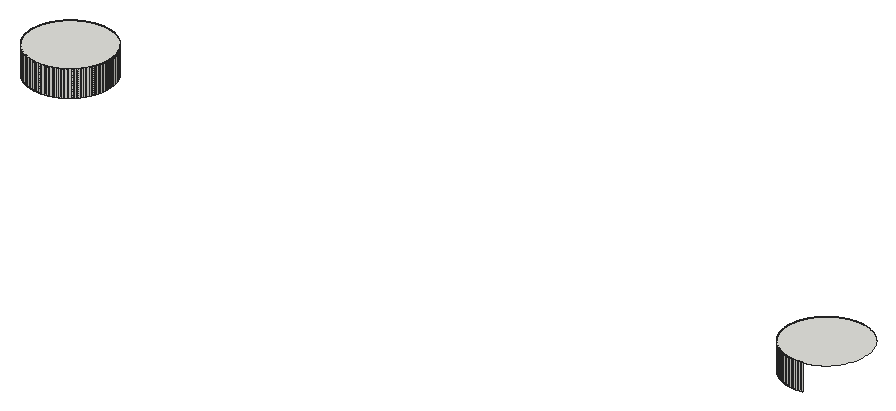
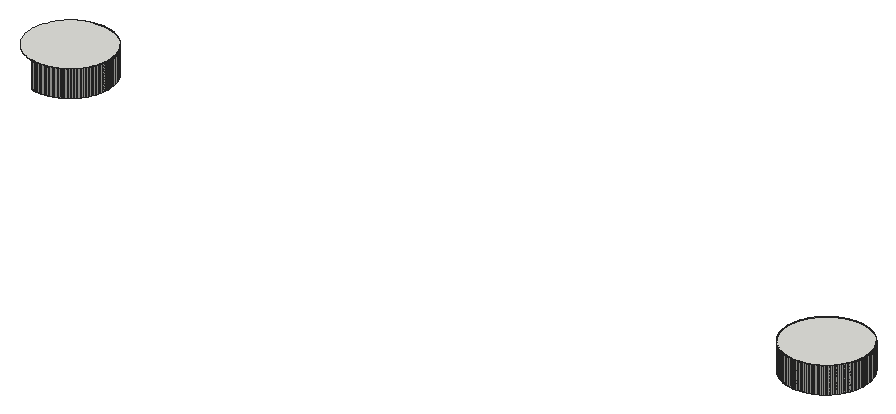
# SketchUp Ruby script. Lengths in inches.
U = 1.inch
M = Sketchup.active_model
def pt(a) = Geom::Point3d.new(a.map { |v| v * U })
def face(e, loops, mat)
  f = e.add_face(loops[0].map { |a| pt(a) })
  loops[1..].each { |l| e.add_face(l.map { |a| pt(a) }).erase! }
  f.material = f.back_material = mat if mat
  f
end
# faces: each face lists its corners as indices into pts; further lists are holes
def faces(e, pts, list, mat = nil) = list.each { |f| face(e, (f[0].is_a?(Array) ? f : [f]).map { |l| l.map { |i| pts[i] } }, mat) }
# xy, xz, yz: faces in a plane at the given z, y or x. An outline is a flat list of corners, or four numbers for a rectangle; further outlines are holes
def ring(l) = l.size == 4 ? [[l[0], l[1]], [l[2], l[1]], [l[2], l[3]], [l[0], l[3]]] : l.each_slice(2).to_a
def flat(e, list, mat, &to3) = list.each { |f| face(e, (f[0].is_a?(Array) ? f : [f]).map { |l| ring(l).map { |u, v| to3.(u, v) } }, mat) }
def xy(e, z, list, mat = nil) = flat(e, list, mat) { |x, y| [x, y, z] }
def xz(e, y, list, mat = nil) = flat(e, list, mat) { |x, z| [x, y, z] }
def yz(e, x, list, mat = nil) = flat(e, list, mat) { |y, z| [x, y, z] }
def lines(e, pts, list) = list.each { |a, b| e.add_line(pt(pts[a]), pt(pts[b])) }
# prism: a flat outline (further loops are holes) pulled along v
def prism(e, loops, v, mat = nil)
  f = face(e, loops, mat); d = Geom::Vector3d.new(v.map { |x| x * U })
  f.pushpull(f.normal.samedirection?(d) ? d.length : -d.length)
end
def box(e, o, s, mat = nil) = prism(e, [[o, [o[0] + s[0], o[1], o[2]], [o[0] + s[0], o[1] + s[1], o[2]], [o[0], o[1] + s[1], o[2]]]], [0, 0, s[2]], mat)
def at(x, y, z, deg = 0) = Geom::Transformation.translation(pt([x, y, z])) * Geom::Transformation.rotation(ORIGIN, Z_AXIS, deg.degrees)
def axes(o, x, y, z) = Geom::Transformation.new([*x, 0, *y, 0, *z, 0, *pt(o).to_a, 1])
def part(name) = M.definitions.add(name)
# library, detail: a bought-in or finely detailed component or shape, given as its bounding box
def library(name, o, s) = part(name).tap { |d| box(d.entities, o, s) }
def detail(e, o, s) = box(e.add_group.entities, o, s)
def put(e, d, t, mat = nil) = e.add_instance(d, t).tap { |i| i.material = mat if mat }
def group(e, t, mat = nil) = e.add_group.tap { |g| g.transformation = t; g.material = mat if mat }.entities
root = M.entities
xy(root,110,[[39.84,175.5,39.76,175.51,39.6875,175.52,39.61,175.53,39.45,175.55,39.375,175.57,39.3,175.58,39.22,175.6,39.15,175.625,39.07,175.65,39,175.67,38.92,175.7,38.71,175.79,38.64,175.83,38.57,175.86,38.43,175.94,38.37,175.98,38.3,176.03,38.24,176.07,38.17,176.12,37.93,176.32,37.88,176.38,37.82,176.43,37.62,176.67,37.57,176.74,37.53,176.8,37.48,176.87,37.44,176.93,37.36,177.07,37.33,177.14,37.29,177.21,37.2,177.42,37.17,177.5,37.15,177.57,37.125,177.65,37.1,177.72,37.08,177.8,37.07,177.875,37.05,177.95,37.03,178.11,37.02,178.1875,37.01,178.26,37,178.34,37,178.66,37.01,178.74,37.02,178.8125,37.03,178.89,37.05,179.05,37.07,179.125,37.08,179.2,37.1,179.28,37.125,179.35,37.15,179.43,37.17,179.5,37.2,179.58,37.29,179.79,37.33,179.86,37.36,179.93,37.44,180.07,37.48,180.13,37.53,180.2,37.57,180.26,37.62,180.33,37.82,180.57,37.88,180.62,37.93,180.68,38.17,180.88,38.24,180.93,38.3,180.97,38.37,181.02,38.43,181.06,38.57,181.14,38.64,181.17,38.71,181.21,38.92,181.3,39,181.33,39.07,181.35,39.15,181.375,39.22,181.4,39.3,181.42,39.375,181.43,39.45,181.45,39.61,181.47,39.6875,181.48,39.76,181.49,39.84,181.5,40.16,181.5,40.24,181.49,40.3125,181.48,40.39,181.47,40.55,181.45,40.625,181.43,40.7,181.42,40.78,181.4,40.85,181.375,40.93,181.35,41,181.33,41.08,181.3,41.29,181.21,41.36,181.17,41.43,181.14,41.57,181.06,41.63,181.02,41.7,180.97,41.76,180.93,41.83,180.88,42.07,180.68,42.12,180.62,42.18,180.57,42.38,180.33,42.43,180.26,42.47,180.2,42.52,180.13,42.56,180.07,42.64,179.93,42.67,179.86,42.71,179.79,42.8,179.58,42.83,179.5,42.85,179.43,42.875,179.35,42.9,179.28,42.92,179.2,42.93,179.125,42.95,179.05,42.97,178.89,42.98,178.8125,42.99,178.74,43,178.66,43,178.34,42.99,178.26,42.98,178.1875,42.97,178.11,42.95,177.95,42.93,177.875,42.92,177.8,42.9,177.72,42.875,177.65,42.85,177.57,42.83,177.5,42.8,177.42,42.71,177.21,42.67,177.14,42.64,177.07,42.56,176.93,42.52,176.87,42.47,176.8,42.43,176.74,42.38,176.67,42.18,176.43,42.12,176.38,42.07,176.32,41.83,176.12,41.76,176.07,41.7,176.03,41.63,175.98,41.57,175.94,41.43,175.86,41.36,175.83,41.29,175.79,41.08,175.7,41,175.67,40.93,175.65,40.85,175.625,40.78,175.6,40.7,175.58,40.625,175.57,40.55,175.55,40.39,175.53,40.3125,175.52,40.24,175.51,40.16,175.5],[98.09,175.5,98.01,175.51,97.9375,175.52,97.86,175.53,97.7,175.55,97.625,175.57,97.55,175.58,97.47,175.6,97.4,175.625,97.32,175.65,97.25,175.67,97.17,175.7,96.96,175.79,96.89,175.83,96.82,175.86,96.68,175.94,96.62,175.98,96.55,176.03,96.49,176.07,96.42,176.12,96.18,176.32,96.13,176.38,96.07,176.43,95.87,176.67,95.82,176.74,95.78,176.8,95.73,176.87,95.69,176.93,95.61,177.07,95.58,177.14,95.54,177.21,95.45,177.42,95.42,177.5,95.4,177.57,95.375,177.65,95.35,177.72,95.33,177.8,95.32,177.875,95.3,177.95,95.28,178.11,95.27,178.1875,95.26,178.26,95.25,178.34,95.25,178.66,95.26,178.74,95.27,178.8125,95.28,178.89,95.3,179.05,95.32,179.125,95.33,179.2,95.35,179.28,95.375,179.35,95.4,179.43,95.42,179.5,95.45,179.58,95.54,179.79,95.58,179.86,95.61,179.93,95.69,180.07,95.73,180.13,95.78,180.2,95.82,180.26,95.87,180.33,96.07,180.57,96.13,180.62,96.18,180.68,96.42,180.88,96.49,180.93,96.55,180.97,96.62,181.02,96.68,181.06,96.82,181.14,96.89,181.17,96.96,181.21,97.17,181.3,97.25,181.33,97.32,181.35,97.4,181.375,97.47,181.4,97.55,181.42,97.625,181.43,97.7,181.45,97.86,181.47,97.9375,181.48,98.01,181.49,98.09,181.5,98.41,181.5,98.49,181.49,98.5625,181.48,98.64,181.47,98.8,181.45,98.875,181.43,98.95,181.42,99.03,181.4,99.1,181.375,99.18,181.35,99.25,181.33,99.33,181.3,99.54,181.21,99.61,181.17,99.68,181.14,99.82,181.06,99.88,181.02,99.95,180.97,100.01,180.93,100.08,180.88,100.32,180.68,100.37,180.62,100.43,180.57,100.63,180.33,100.68,180.26,100.72,180.2,100.77,180.13,100.81,180.07,100.89,179.93,100.92,179.86,100.96,179.79,101.05,179.58,101.08,179.5,101.1,179.43,101.125,179.35,101.15,179.28,101.17,179.2,101.18,179.125,101.2,179.05,101.22,178.89,101.23,178.8125,101.24,178.74,101.25,178.66,101.25,178.34,101.24,178.26,101.23,178.1875,101.22,178.11,101.2,177.95,101.18,177.875,101.17,177.8,101.15,177.72,101.125,177.65,101.1,177.57,101.08,177.5,101.05,177.42,100.96,177.21,100.92,177.14,100.89,177.07,100.81,176.93,100.77,176.87,100.72,176.8,100.68,176.74,100.63,176.67,100.43,176.43,100.37,176.38,100.32,176.32,100.08,176.12,100.01,176.07,99.95,176.03,99.88,175.98,99.82,175.94,99.68,175.86,99.61,175.83,99.54,175.79,99.33,175.7,99.25,175.67,99.18,175.65,99.1,175.625,99.03,175.6,98.95,175.58,98.875,175.57,98.8,175.55,98.64,175.53,98.5625,175.52,98.49,175.51,98.41,175.5]])
xz(root,175.5,[[39.84,108,39.92,110],[39.92,108,40,110],[40,108,40.08,110],[40.08,108,40.16,110],[98.09,108,98.17,110],
  [98.17,108,98.25,110],[98.25,108,98.33,110],[98.33,108,98.41,110]])
xz(root,181.5,[[39.84,108,39.92,110],[39.92,108,40,110],[40,108,40.08,110],[40.08,108,40.16,110],[98.09,108,98.17,110],
  [98.17,108,98.25,110],[98.25,108,98.33,110],[98.33,108,98.41,110]])
yz(root,37,[[178.34,108,178.42,110],[178.42,108,178.5,110],[178.5,108,178.58,110],[178.58,108,178.66,110]])
yz(root,43,[[178.34,108,178.42,110],[178.42,108,178.5,110],[178.5,108,178.58,110],[178.58,108,178.66,110]])
yz(root,95.25,[[178.34,108,178.42,110],[178.42,108,178.5,110],[178.5,108,178.58,110],[178.58,108,178.66,110]])
p = [[39.53,175.54,108],[39.45,175.55,108],[39.45,175.55,110],[39.53,175.54,110],[39.61,175.53,108],[39.61,175.53,110],
  [39.6875,175.52,108],[39.6875,175.52,110],[39.76,175.51,108],[39.76,175.51,110],[39.84,175.5,108],[39.84,175.5,110],
  [40.24,175.51,108],[40.16,175.5,108],[40.16,175.5,110],[40.24,175.51,110],[40.3125,175.52,108],[40.3125,175.52,110],
  [40.39,175.53,108],[40.39,175.53,110],[40.47,175.54,108],[40.47,175.54,110],[40.55,175.55,108],[40.55,175.55,110],
  [97.78,175.54,108],[97.7,175.55,108],[97.7,175.55,110],[97.78,175.54,110],[97.86,175.53,108],[97.86,175.53,110],
  [97.9375,175.52,108],[97.9375,175.52,110],[98.01,175.51,108],[98.01,175.51,110],[98.09,175.5,108],[98.09,175.5,110],
  [98.49,175.51,108],[98.41,175.5,108],[98.41,175.5,110],[98.49,175.51,110],[98.5625,175.52,108],[98.5625,175.52,110],
  [98.64,175.53,108],[98.64,175.53,110],[98.72,175.54,108],[98.72,175.54,110],[98.8,175.55,108],[98.8,175.55,110],
  [39.07,175.65,108],[39,175.67,108],[39,175.67,110],[39.07,175.65,110],[39.15,175.625,108],[39.15,175.625,110],
  [39.22,175.6,108],[39.22,175.6,110],[39.3,175.58,108],[39.3,175.58,110],[39.375,175.57,108],[39.375,175.57,110],
  [40.625,175.57,108],[40.625,175.57,110],[40.7,175.58,108],[40.7,175.58,110],[40.78,175.6,108],[40.78,175.6,110],
  [40.85,175.625,108],[40.85,175.625,110],[40.93,175.65,108],[40.93,175.65,110],[41,175.67,108],[41,175.67,110],
  [97.32,175.65,108],[97.25,175.67,108],[97.25,175.67,110],[97.32,175.65,110],[97.4,175.625,108],[97.4,175.625,110],
  [97.47,175.6,108],[97.47,175.6,110],[97.55,175.58,108],[97.55,175.58,110],[97.625,175.57,108],[97.625,175.57,110],
  [38.85,175.73,108],[38.78,175.76,108],[38.78,175.76,110],[38.85,175.73,110],[38.92,175.7,108],[38.92,175.7,110],
  [41.08,175.7,108],[41.08,175.7,110],[41.15,175.73,108],[41.15,175.73,110],[41.22,175.76,108],[41.22,175.76,110],
  [97.1,175.73,108],[97.03,175.76,108],[97.03,175.76,110],[97.1,175.73,110],[97.17,175.7,108],[97.17,175.7,110],
  [38.64,175.83,108],[38.57,175.86,108],[38.57,175.86,110],[38.64,175.83,110],[38.71,175.79,108],[38.71,175.79,110],
  [41.29,175.79,108],[41.29,175.79,110],[41.36,175.83,108],[41.36,175.83,110],[41.43,175.86,108],[41.43,175.86,110],
  [96.89,175.83,108],[96.82,175.86,108],[96.82,175.86,110],[96.89,175.83,110],[96.96,175.79,108],[96.96,175.79,110],
  [38.43,175.94,108],[38.37,175.98,108],[38.37,175.98,110],[38.43,175.94,110],[38.5,175.9,108],[38.5,175.9,110],
  [41.5,175.9,108],[41.5,175.9,110],[41.57,175.94,108],[41.57,175.94,110],[41.63,175.98,108],[41.63,175.98,110],
  [96.68,175.94,108],[96.62,175.98,108],[96.62,175.98,110],[96.68,175.94,110],[96.75,175.9,108],[96.75,175.9,110],
  [38.3,176.03,108],[38.24,176.07,108],[38.24,176.07,110],[38.3,176.03,110],[41.7,176.03,108],[41.7,176.03,110],
  [41.76,176.07,108],[41.76,176.07,110],[96.55,176.03,108],[96.49,176.07,108],[96.49,176.07,110],[96.55,176.03,110],
  [38.17,176.12,108],[38.11,176.17,108],[38.11,176.17,110],[38.17,176.12,110],[41.83,176.12,108],[41.83,176.12,110],
  [41.89,176.17,108],[41.89,176.17,110],[96.42,176.12,108],[96.36,176.17,108],[96.36,176.17,110],[96.42,176.12,110],
  [38.05,176.22,108],[37.99,176.27,108],[37.99,176.27,110],[38.05,176.22,110],[41.95,176.22,108],[41.95,176.22,110],
  [42.01,176.27,108],[42.01,176.27,110],[96.3,176.22,108],[96.24,176.27,108],[96.24,176.27,110],[96.3,176.22,110],
  [37.93,176.32,108],[37.88,176.38,108],[37.88,176.38,110],[37.93,176.32,110],[42.07,176.32,108],[42.07,176.32,110],
  [42.12,176.38,108],[42.12,176.38,110],[96.18,176.32,108],[96.13,176.38,108],[96.13,176.38,110],[96.18,176.32,110],
  [37.82,176.43,108],[37.77,176.49,108],[37.77,176.49,110],[37.82,176.43,110],[42.18,176.43,108],[42.18,176.43,110],
  [42.23,176.49,108],[42.23,176.49,110],[96.07,176.43,108],[96.02,176.49,108],[96.02,176.49,110],[96.07,176.43,110],
  [37.72,176.55,108],[37.72,176.55,110],[42.28,176.55,108],[42.28,176.55,110],[95.97,176.55,108],[95.97,176.55,110],
  [37.67,176.61,108],[37.62,176.67,108],[37.62,176.67,110],[37.67,176.61,110],[42.33,176.61,108],[42.33,176.61,110],
  [42.38,176.67,108],[42.38,176.67,110],[95.92,176.61,108],[95.87,176.67,108],[95.87,176.67,110],[95.92,176.61,110],
  [37.57,176.74,108],[37.53,176.8,108],[37.53,176.8,110],[37.57,176.74,110],[42.43,176.74,108],[42.43,176.74,110],
  [42.47,176.8,108],[42.47,176.8,110],[95.82,176.74,108],[95.78,176.8,108],[95.78,176.8,110],[95.82,176.74,110],
  [37.48,176.87,108],[37.48,176.87,110],[42.52,176.87,108],[42.52,176.87,110],[95.73,176.87,108],[95.73,176.87,110],
  [37.44,176.93,108],[37.4,177,108],[37.4,177,110],[37.44,176.93,110],[42.56,176.93,108],[42.56,176.93,110],
  [42.6,177,108],[42.6,177,110],[95.69,176.93,108],[95.65,177,108],[95.65,177,110],[95.69,176.93,110],
  [37.36,177.07,108],[37.36,177.07,110],[42.64,177.07,108],[42.64,177.07,110],[95.61,177.07,108],[95.61,177.07,110],
  [37.33,177.14,108],[37.29,177.21,108],[37.29,177.21,110],[37.33,177.14,110],[42.67,177.14,108],[42.67,177.14,110],
  [42.71,177.21,108],[42.71,177.21,110],[95.58,177.14,108],[95.54,177.21,108],[95.54,177.21,110],[95.58,177.14,110],
  [37.26,177.28,108],[37.26,177.28,110],[42.74,177.28,108],[42.74,177.28,110],[95.51,177.28,108],[95.51,177.28,110],
  [37.23,177.35,108],[37.23,177.35,110],[42.77,177.35,108],[42.77,177.35,110],[95.48,177.35,108],[95.48,177.35,110],
  [37.2,177.42,108],[37.17,177.5,108],[37.17,177.5,110],[37.2,177.42,110],[42.8,177.42,108],[42.8,177.42,110],
  [42.83,177.5,108],[42.83,177.5,110],[95.45,177.42,108],[95.42,177.5,108],[95.42,177.5,110],[95.45,177.42,110],
  [37.15,177.57,108],[37.15,177.57,110],[42.85,177.57,108],[42.85,177.57,110],[95.4,177.57,108],[95.4,177.57,110],
  [37.125,177.65,108],[37.1,177.72,108],[37.1,177.72,110],[37.125,177.65,110],[42.875,177.65,108],[42.875,177.65,110],
  [42.9,177.72,108],[42.9,177.72,110],[95.375,177.65,108],[95.35,177.72,108],[95.35,177.72,110],[95.375,177.65,110],
  [37.08,177.8,108],[37.08,177.8,110],[42.92,177.8,108],[42.92,177.8,110],[95.33,177.8,108],[95.33,177.8,110],
  [37.07,177.875,108],[37.07,177.875,110],[42.93,177.875,108],[42.93,177.875,110],[95.32,177.875,108],[95.32,177.875,110],
  [37.05,177.95,108],[37.05,177.95,110],[42.95,177.95,108],[42.95,177.95,110],[95.3,177.95,108],[95.3,177.95,110],
  [37.04,178.03,108],[37.03,178.11,108],[37.03,178.11,110],[37.04,178.03,110],[42.96,178.03,108],[42.96,178.03,110],
  [42.97,178.11,108],[42.97,178.11,110],[95.29,178.03,108],[95.28,178.11,108],[95.28,178.11,110],[95.29,178.03,110],
  [37.02,178.1875,108],[37.02,178.1875,110],[42.98,178.1875,108],[42.98,178.1875,110],[95.27,178.1875,108],[95.27,178.1875,110],
  [37.01,178.26,108],[37.01,178.26,110],[42.99,178.26,108],[42.99,178.26,110],[95.26,178.26,108],[95.26,178.26,110],
  [37,178.34,108],[37,178.34,110],[43,178.34,108],[43,178.34,110],[95.25,178.34,108],[95.25,178.34,110],
  [37,178.66,108],[37.01,178.74,108],[37.01,178.74,110],[37,178.66,110],[37.02,178.8125,108],[37.02,178.8125,110],
  [42.98,178.8125,108],[42.99,178.74,108],[42.99,178.74,110],[42.98,178.8125,110],[43,178.66,108],[43,178.66,110],
  [95.25,178.66,108],[95.26,178.74,108],[95.26,178.74,110],[95.25,178.66,110],[95.27,178.8125,108],[95.27,178.8125,110],
  [37.03,178.89,108],[37.03,178.89,110],[42.97,178.89,108],[42.97,178.89,110],[95.28,178.89,108],[95.28,178.89,110],
  [37.04,178.97,108],[37.04,178.97,110],[42.96,178.97,108],[42.96,178.97,110],[95.29,178.97,108],[95.29,178.97,110],
  [37.05,179.05,108],[37.05,179.05,110],[37.07,179.125,108],[37.07,179.125,110],[42.93,179.125,108],[42.95,179.05,108],
  [42.95,179.05,110],[42.93,179.125,110],[95.3,179.05,108],[95.3,179.05,110],[95.32,179.125,108],[95.32,179.125,110],
  [37.08,179.2,108],[37.08,179.2,110],[42.92,179.2,108],[42.92,179.2,110],[95.33,179.2,108],[95.33,179.2,110],
  [37.1,179.28,108],[37.1,179.28,110],[42.9,179.28,108],[42.9,179.28,110],[95.35,179.28,108],[95.35,179.28,110],
  [37.125,179.35,108],[37.125,179.35,110],[42.875,179.35,108],[42.875,179.35,110],[95.375,179.35,108],[95.375,179.35,110],
  [37.15,179.43,108],[37.15,179.43,110],[37.17,179.5,108],[37.17,179.5,110],[42.83,179.5,108],[42.85,179.43,108],
  [42.85,179.43,110],[42.83,179.5,110],[95.4,179.43,108],[95.4,179.43,110],[95.42,179.5,108],[95.42,179.5,110],
  [37.2,179.58,108],[37.2,179.58,110],[42.8,179.58,108],[42.8,179.58,110],[95.45,179.58,108],[95.45,179.58,110],
  [37.23,179.65,108],[37.23,179.65,110],[37.26,179.72,108],[37.26,179.72,110],[42.74,179.72,108],[42.77,179.65,108],
  [42.77,179.65,110],[42.74,179.72,110],[95.48,179.65,108],[95.48,179.65,110],[95.51,179.72,108],[95.51,179.72,110],
  [37.29,179.79,108],[37.29,179.79,110],[42.71,179.79,108],[42.71,179.79,110],[95.54,179.79,108],[95.54,179.79,110],
  [37.33,179.86,108],[37.33,179.86,110],[42.67,179.86,108],[42.67,179.86,110],[95.58,179.86,108],[95.58,179.86,110],
  [37.36,179.93,108],[37.36,179.93,110],[37.4,180,108],[37.4,180,110],[42.6,180,108],[42.64,179.93,108],
  [42.64,179.93,110],[42.6,180,110],[95.61,179.93,108],[95.61,179.93,110],[95.65,180,108],[95.65,180,110],
  [37.44,180.07,108],[37.44,180.07,110],[42.56,180.07,108],[42.56,180.07,110],[95.69,180.07,108],[95.69,180.07,110],
  [37.48,180.13,108],[37.48,180.13,110],[37.53,180.2,108],[37.53,180.2,110],[42.47,180.2,108],[42.52,180.13,108],
  [42.52,180.13,110],[42.47,180.2,110],[95.73,180.13,108],[95.73,180.13,110],[95.78,180.2,108],[95.78,180.2,110],
  [37.57,180.26,108],[37.57,180.26,110],[42.43,180.26,108],[42.43,180.26,110],[95.82,180.26,108],[95.82,180.26,110],
  [37.62,180.33,108],[37.62,180.33,110],[37.67,180.39,108],[37.67,180.39,110],[42.33,180.39,108],[42.38,180.33,108],
  [42.38,180.33,110],[42.33,180.39,110],[95.87,180.33,108],[95.87,180.33,110],[95.92,180.39,108],[95.92,180.39,110],
  [37.72,180.45,108],[37.72,180.45,110],[37.77,180.51,108],[37.77,180.51,110],[42.23,180.51,108],[42.28,180.45,108],
  [42.28,180.45,110],[42.23,180.51,110],[95.97,180.45,108],[95.97,180.45,110],[96.02,180.51,108],[96.02,180.51,110],
  [37.82,180.57,108],[37.82,180.57,110],[42.18,180.57,108],[42.18,180.57,110],[96.07,180.57,108],[96.07,180.57,110],
  [37.88,180.62,108],[37.88,180.62,110],[37.93,180.68,108],[37.93,180.68,110],[42.07,180.68,108],[42.12,180.62,108],
  [42.12,180.62,110],[42.07,180.68,110],[96.13,180.62,108],[96.13,180.62,110],[96.18,180.68,108],[96.18,180.68,110],
  [37.99,180.73,108],[37.99,180.73,110],[38.05,180.78,108],[38.05,180.78,110],[41.95,180.78,108],[42.01,180.73,108],
  [42.01,180.73,110],[41.95,180.78,110],[96.24,180.73,108],[96.24,180.73,110],[96.3,180.78,108],[96.3,180.78,110],
  [38.11,180.83,108],[38.11,180.83,110],[38.17,180.88,108],[38.17,180.88,110],[41.83,180.88,108],[41.89,180.83,108],
  [41.89,180.83,110],[41.83,180.88,110],[96.36,180.83,108],[96.36,180.83,110],[96.42,180.88,108],[96.42,180.88,110],
  [38.24,180.93,108],[38.24,180.93,110],[38.3,180.97,108],[38.3,180.97,110],[41.7,180.97,108],[41.76,180.93,108],
  [41.76,180.93,110],[41.7,180.97,110],[96.49,180.93,108],[96.49,180.93,110],[96.55,180.97,108],[96.55,180.97,110],
  [38.37,181.02,108],[38.37,181.02,110],[38.43,181.06,108],[38.43,181.06,110],[41.57,181.06,108],[41.63,181.02,108],
  [41.63,181.02,110],[41.57,181.06,110],[96.62,181.02,108],[96.62,181.02,110],[96.68,181.06,108],[96.68,181.06,110],
  [38.5,181.1,108],[38.5,181.1,110],[38.57,181.14,108],[38.57,181.14,110],[38.64,181.17,108],[38.64,181.17,110],
  [41.36,181.17,108],[41.43,181.14,108],[41.43,181.14,110],[41.36,181.17,110],[41.5,181.1,108],[41.5,181.1,110],
  [96.75,181.1,108],[96.75,181.1,110],[96.82,181.14,108],[96.82,181.14,110],[96.89,181.17,108],[96.89,181.17,110],
  [38.71,181.21,108],[38.71,181.21,110],[38.78,181.24,108],[38.78,181.24,110],[38.85,181.27,108],[38.85,181.27,110],
  [41.15,181.27,108],[41.22,181.24,108],[41.22,181.24,110],[41.15,181.27,110],[41.29,181.21,108],[41.29,181.21,110],
  [96.96,181.21,108],[96.96,181.21,110],[97.03,181.24,108],[97.03,181.24,110],[97.1,181.27,108],[97.1,181.27,110],
  [38.92,181.3,108],[38.92,181.3,110],[39,181.33,108],[39,181.33,110],[39.07,181.35,108],[39.07,181.35,110],
  [40.93,181.35,108],[41,181.33,108],[41,181.33,110],[40.93,181.35,110],[41.08,181.3,108],[41.08,181.3,110],
  [97.17,181.3,108],[97.17,181.3,110],[97.25,181.33,108],[97.25,181.33,110],[97.32,181.35,108],[97.32,181.35,110],
  [39.15,181.375,108],[39.15,181.375,110],[39.22,181.4,108],[39.22,181.4,110],[39.3,181.42,108],[39.3,181.42,110],
  [39.375,181.43,108],[39.375,181.43,110],[39.45,181.45,108],[39.45,181.45,110],[39.53,181.46,108],[39.53,181.46,110],
  [40.47,181.46,108],[40.55,181.45,108],[40.55,181.45,110],[40.47,181.46,110],[40.625,181.43,108],[40.625,181.43,110],
  [40.7,181.42,108],[40.7,181.42,110],[40.78,181.4,108],[40.78,181.4,110],[40.85,181.375,108],[40.85,181.375,110],
  [97.4,181.375,108],[97.4,181.375,110],[97.47,181.4,108],[97.47,181.4,110],[97.55,181.42,108],[97.55,181.42,110],
  [97.625,181.43,108],[97.625,181.43,110],[97.7,181.45,108],[97.7,181.45,110],[97.78,181.46,108],[97.78,181.46,110],
  [98.72,181.46,108],[98.8,181.45,108],[98.8,181.45,110],[98.72,181.46,110],[98.875,181.43,108],[98.875,181.43,110],
  [39.61,181.47,108],[39.61,181.47,110],[39.6875,181.48,108],[39.6875,181.48,110],[39.76,181.49,108],[39.76,181.49,110],
  [39.84,181.5,108],[39.84,181.5,110],[40.16,181.5,108],[40.24,181.49,108],[40.24,181.49,110],[40.16,181.5,110],
  [40.3125,181.48,108],[40.3125,181.48,110],[40.39,181.47,108],[40.39,181.47,110],[97.86,181.47,108],[97.86,181.47,110],
  [97.9375,181.48,108],[97.9375,181.48,110],[98.01,181.49,108],[98.01,181.49,110],[98.09,181.5,108],[98.09,181.5,110],
  [98.41,181.5,108],[98.49,181.49,108],[98.49,181.49,110],[98.41,181.5,110],[98.5625,181.48,108],[98.5625,181.48,110],
  [98.64,181.47,108],[98.64,181.47,110]]
faces(root,p,[[0,1,2,3],[4,0,3,5],[6,4,5,7],[8,6,7,9],[10,8,9,11],[12,13,14,15],[16,12,15,17],[18,16,17,19],
  [20,18,19,21],[22,20,21,23],[24,25,26,27],[28,24,27,29],[30,28,29,31],[32,30,31,33],[34,32,33,35],[36,37,38,39],
  [40,36,39,41],[42,40,41,43],[44,42,43,45],[46,44,45,47],[48,49,50,51],[52,48,51,53],[54,52,53,55],[56,54,55,57],
  [58,56,57,59],[1,58,59,2],[60,22,23,61],[62,60,61,63],[64,62,63,65],[66,64,65,67],[68,66,67,69],[70,68,69,71],
  [72,73,74,75],[76,72,75,77],[78,76,77,79],[80,78,79,81],[82,80,81,83],[25,82,83,26],[84,85,86,87],[88,84,87,89],
  [49,88,89,50],[90,70,71,91],[92,90,91,93],[94,92,93,95],[96,97,98,99],[100,96,99,101],[73,100,101,74],[102,103,104,105],
  [106,102,105,107],[85,106,107,86],[108,94,95,109],[110,108,109,111],[112,110,111,113],[114,115,116,117],[118,114,117,119],[97,118,119,98],
  [120,121,122,123],[124,120,123,125],[103,124,125,104],[126,112,113,127],[128,126,127,129],[130,128,129,131],[132,133,134,135],[136,132,135,137],
  [115,136,137,116],[138,139,140,141],[121,138,141,122],[142,130,131,143],[144,142,143,145],[146,147,148,149],[133,146,149,134],[150,151,152,153],
  [139,150,153,140],[154,144,145,155],[156,154,155,157],[158,159,160,161],[147,158,161,148],[162,163,164,165],[151,162,165,152],[166,156,157,167],
  [168,166,167,169],[170,171,172,173],[159,170,173,160],[174,175,176,177],[163,174,177,164],[178,168,169,179],[180,178,179,181],[182,183,184,185],
  [171,182,185,172],[186,187,188,189],[175,186,189,176],[190,180,181,191],[192,190,191,193],[194,195,196,197],[183,194,197,184],[187,198,199,188],
  [200,192,193,201],[195,202,203,196],[204,205,206,207],[198,204,207,199],[208,200,201,209],[210,208,209,211],[212,213,214,215],[202,212,215,203],
  [216,217,218,219],[205,216,219,206],[220,210,211,221],[222,220,221,223],[224,225,226,227],[213,224,227,214],[217,228,229,218],[230,222,223,231],
  [225,232,233,226],[234,235,236,237],[228,234,237,229],[238,230,231,239],[240,238,239,241],[242,243,244,245],[232,242,245,233],[235,246,247,236],
  [248,240,241,249],[243,250,251,244],[252,253,254,255],[246,252,255,247],[256,248,249,257],[258,256,257,259],[260,261,262,263],[250,260,263,251],
  [253,264,265,254],[266,258,259,267],[261,268,269,262],[264,270,271,265],[272,266,267,273],[268,274,275,269],[276,277,278,279],[270,276,279,271],
  [280,272,273,281],[282,280,281,283],[284,285,286,287],[274,284,287,275],[277,288,289,278],[290,282,283,291],[285,292,293,286],[294,295,296,297],
  [288,294,297,289],[298,290,291,299],[300,298,299,301],[302,303,304,305],[292,302,305,293],[295,306,307,296],[308,300,301,309],[303,310,311,304],
  [306,312,313,307],[314,308,309,315],[310,316,317,311],[312,318,319,313],[320,314,315,321],[316,322,323,317],[324,325,326,327],[318,324,327,319],
  [328,320,321,329],[330,328,329,331],[332,333,334,335],[322,332,335,323],[325,336,337,326],[338,330,331,339],[333,340,341,334],[336,342,343,337],
  [344,338,339,345],[340,346,347,341],[342,348,349,343],[350,344,345,351],[346,352,353,347],[354,355,356,357],[355,358,359,356],[360,361,362,363],
  [361,364,365,362],[366,367,368,369],[367,370,371,368],[358,372,373,359],[374,360,363,375],[370,376,377,371],[372,378,379,373],[380,374,375,381],
  [376,382,383,377],[378,384,385,379],[384,386,387,385],[388,389,390,391],[389,380,381,390],[382,392,393,383],[392,394,395,393],[386,396,397,387],
  [398,388,391,399],[394,400,401,395],[396,402,403,397],[404,398,399,405],[400,406,407,401],[402,408,409,403],[410,404,405,411],[406,412,413,407],
  [408,414,415,409],[414,416,417,415],[418,419,420,421],[419,410,411,420],[412,422,423,413],[422,424,425,423],[416,426,427,417],[428,418,421,429],
  [424,430,431,425],[426,432,433,427],[432,434,435,433],[436,437,438,439],[437,428,429,438],[430,440,441,431],[440,442,443,441],[434,444,445,435],
  [446,436,439,447],[442,448,449,443],[444,450,451,445],[452,446,447,453],[448,454,455,449],[450,456,457,451],[456,458,459,457],[460,461,462,463],
  [461,452,453,462],[454,464,465,455],[464,466,467,465],[458,468,469,459],[470,460,463,471],[466,472,473,467],[468,474,475,469],[474,476,477,475],
  [478,479,480,481],[479,470,471,480],[472,482,483,473],[482,484,485,483],[476,486,487,477],[488,478,481,489],[484,490,491,485],[486,492,493,487],
  [492,494,495,493],[496,497,498,499],[497,488,489,498],[490,500,501,491],[500,502,503,501],[494,504,505,495],[504,506,507,505],[508,509,510,511],
  [509,496,499,510],[502,512,513,503],[512,514,515,513],[506,516,517,507],[518,508,511,519],[514,520,521,515],[516,522,523,517],[522,524,525,523],
  [526,527,528,529],[527,518,519,528],[520,530,531,521],[530,532,533,531],[524,534,535,525],[534,536,537,535],[538,539,540,541],[539,526,529,540],
  [532,542,543,533],[542,544,545,543],[536,546,547,537],[546,548,549,547],[550,551,552,553],[551,538,541,552],[544,554,555,545],[554,556,557,555],
  [548,558,559,549],[558,560,561,559],[562,563,564,565],[563,550,553,564],[556,566,567,557],[566,568,569,567],[560,570,571,561],[570,572,573,571],
  [574,575,576,577],[575,562,565,576],[568,578,579,569],[578,580,581,579],[572,582,583,573],[582,584,585,583],[584,586,587,585],[588,589,590,591],
  [589,592,593,590],[592,574,577,593],[580,594,595,581],[594,596,597,595],[596,598,599,597],[586,600,601,587],[600,602,603,601],[602,604,605,603],
  [606,607,608,609],[607,610,611,608],[610,588,591,611],[598,612,613,599],[612,614,615,613],[614,616,617,615],[604,618,619,605],[618,620,621,619],
  [620,622,623,621],[624,625,626,627],[625,628,629,626],[628,606,609,629],[616,630,631,617],[630,632,633,631],[632,634,635,633],[622,636,637,623],
  [636,638,639,637],[638,640,641,639],[640,642,643,641],[642,644,645,643],[644,646,647,645],[648,649,650,651],[649,652,653,650],[652,654,655,653],
  [654,656,657,655],[656,658,659,657],[658,624,627,659],[634,660,661,635],[660,662,663,661],[662,664,665,663],[664,666,667,665],[666,668,669,667],
  [668,670,671,669],[672,673,674,675],[673,676,677,674],[646,678,679,647],[678,680,681,679],[680,682,683,681],[682,684,685,683],[686,687,688,689],
  [687,690,691,688],[690,692,693,691],[692,648,651,693],[670,694,695,671],[694,696,697,695],[696,698,699,697],[698,700,701,699],[702,703,704,705],
  [703,706,707,704],[706,708,709,707],[708,672,675,709]])
